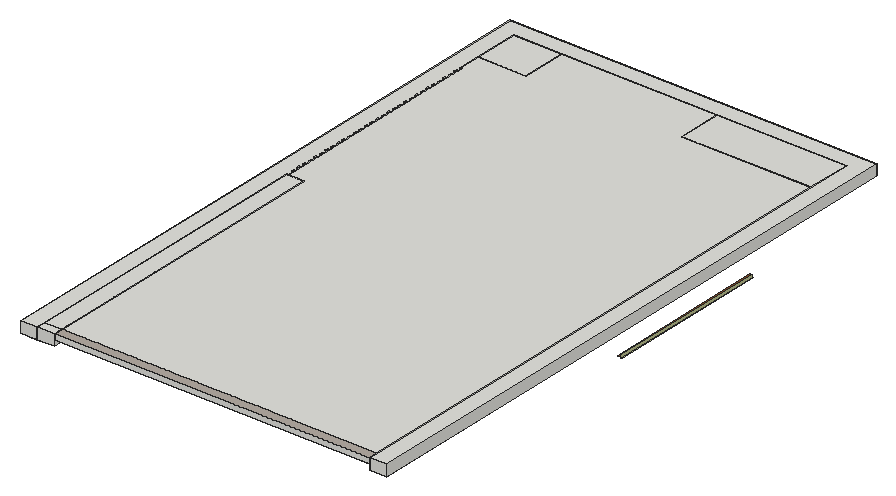
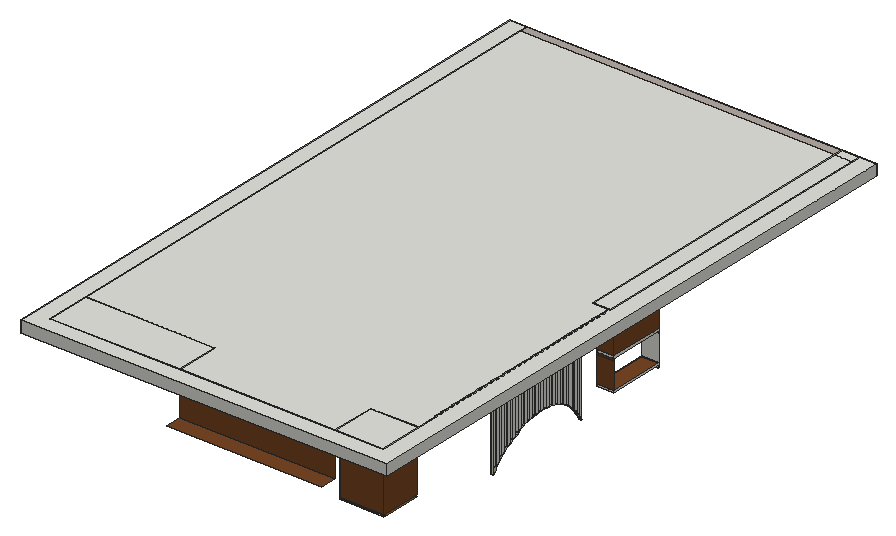
# SketchUp Ruby script. Lengths in inches.
U = 1.inch
M = Sketchup.active_model
def pt(a) = Geom::Point3d.new(a.map { |v| v * U })
def face(e, loops, mat)
  f = e.add_face(loops[0].map { |a| pt(a) })
  loops[1..].each { |l| e.add_face(l.map { |a| pt(a) }).erase! }
  f.material = f.back_material = mat if mat
  f
end
# faces: each face lists its corners as indices into pts; further lists are holes
def faces(e, pts, list, mat = nil) = list.each { |f| face(e, (f[0].is_a?(Array) ? f : [f]).map { |l| l.map { |i| pts[i] } }, mat) }
# xy, xz, yz: faces in a plane at the given z, y or x. An outline is a flat list of corners, or four numbers for a rectangle; further outlines are holes
def ring(l) = l.size == 4 ? [[l[0], l[1]], [l[2], l[1]], [l[2], l[3]], [l[0], l[3]]] : l.each_slice(2).to_a
def flat(e, list, mat, &to3) = list.each { |f| face(e, (f[0].is_a?(Array) ? f : [f]).map { |l| ring(l).map { |u, v| to3.(u, v) } }, mat) }
def xy(e, z, list, mat = nil) = flat(e, list, mat) { |x, y| [x, y, z] }
def xz(e, y, list, mat = nil) = flat(e, list, mat) { |x, z| [x, y, z] }
def yz(e, x, list, mat = nil) = flat(e, list, mat) { |y, z| [x, y, z] }
def lines(e, pts, list) = list.each { |a, b| e.add_line(pt(pts[a]), pt(pts[b])) }
# prism: a flat outline (further loops are holes) pulled along v
def prism(e, loops, v, mat = nil)
  f = face(e, loops, mat); d = Geom::Vector3d.new(v.map { |x| x * U })
  f.pushpull(f.normal.samedirection?(d) ? d.length : -d.length)
end
def box(e, o, s, mat = nil) = prism(e, [[o, [o[0] + s[0], o[1], o[2]], [o[0] + s[0], o[1] + s[1], o[2]], [o[0], o[1] + s[1], o[2]]]], [0, 0, s[2]], mat)
def at(x, y, z, deg = 0) = Geom::Transformation.translation(pt([x, y, z])) * Geom::Transformation.rotation(ORIGIN, Z_AXIS, deg.degrees)
def axes(o, x, y, z) = Geom::Transformation.new([*x, 0, *y, 0, *z, 0, *pt(o).to_a, 1])
def part(name) = M.definitions.add(name)
# library, detail: a bought-in or finely detailed component or shape, given as its bounding box
def library(name, o, s) = part(name).tap { |d| box(d.entities, o, s) }
def detail(e, o, s) = box(e.add_group.entities, o, s)
def put(e, d, t, mat = nil) = e.add_instance(d, t).tap { |i| i.material = mat if mat }
def group(e, t, mat = nil) = e.add_group.tap { |g| g.transformation = t; g.material = mat if mat }.entities
root = M.entities
M.materials.add("Emissive").color = [188, 193, 143]
M.materials.add("Generic\#1").color = [209, 204, 204]
M.materials.add("Tiles L01 200cm").color = [180, 171, 163]
M.materials.add("[Wood Veneer 01]").color = [120, 70, 37]
c1 = library("Books 297 001 004",[-3.55,-2.96,-0.03],[7.44,5.56,6.72])
c2 = library("Tlon Light 1950 Ceiling 152 010",[-38.39,-38.39,-3.78],[76.78,76.78,3.41])
xy(root,83.25,[[9,135.6,18.5,135.64]])
xy(root,84.82,[[9,135.65,10,165.95]],"Emissive")
xy(root,84.82,[[10,135.65,18.5,165.95]],"[Wood Veneer 01]")
xy(root,85.69,[[9,135.6,18.5,135.64]])
xy(root,85.69,[[9,135.64,18.5,165.95]],"[Wood Veneer 01]")
xy(root,92,[[10.03,319.1875,34,320.1875]],"Emissive")
xy(root,92,[[10.03,298.1875,34,319.1875]],"[Wood Veneer 01]")
xy(root,93,[[10,298.1875,34,320.1875]],"[Wood Veneer 01]")
xy(root,97.62,[[8.625,217.16,9.8125,217.65],[8.625,217.65,9.8125,217.68]],"Emissive")
xy(root,99.15,[[188.1875,170.86,189,259.23]],"Emissive")
xy(root,100.27,[[187.125,169.73,188.1875,259.23]],"[Wood Veneer 01]")
xy(root,101.13,[[9,135.6,10,165.91]],"Emissive")
xy(root,101.13,[[10,135.6,18.5,165.91]],"[Wood Veneer 01]")
xy(root,102.44,[[9,135.6,18.5,165.91]],"[Wood Veneer 01]")
xy(root,102.58,[[35,322.1875,119,331.1875]],"[Wood Veneer 01]")
xy(root,115,[[10,319.1875,34,320.1875]],"Emissive")
xy(root,115,[[10,298.1875,34,319.1875]],"[Wood Veneer 01]")
xy(root,116,[[9,298.1875,35,322.1875]])
xy(root,117.41,[[9,135.78,10,166.08]],"Emissive")
xy(root,117.41,[[10,135.78,18.5,166.08]],"[Wood Veneer 01]")
xy(root,120,[[0,0,0,331.1875,198,331.1875,198,0,189,0,189,322.1875,9,322.1875,9,285.93,9.8125,285.93,9.8125,283.51,9,283.51,9,282.14,9.8125,282.14,9.8125,279.71,9,279.71,9,278.35,9.8125,278.35,9.8125,275.92,9,275.92,9,274.56,9.8125,274.56,9.8125,272.13,9,272.13,9,270.77,9.8125,270.77,9.8125,268.34,9,268.34,9,266.97,9.8125,266.97,9.8125,264.55,9,264.55,9,263.18,9.8125,263.18,9.8125,260.76,9,260.76,9,259.39,9.8125,259.39,9.8125,256.96,9,256.96,9,255.6,9.8125,255.6,9.8125,253.17,9,253.17,9,251.81,9.8125,251.81,9.8125,249.38,9,249.38,9,248.02,9.8125,248.02,9.8125,245.59,9,245.59,9,244.22,9.8125,244.22,9.8125,241.8,9,241.8,9,240.43,9.8125,240.43,9.8125,238.01,9,238.01,9,236.64,9.8125,236.64,9.8125,234.21,9,234.21,9,232.85,9.8125,232.85,9.8125,230.42,9,230.42,9,229.06,9.8125,229.06,9.8125,226.63,9,226.63,9,225.27,9.8125,225.27,9.8125,222.84,9,222.84,9,221.47,9.8125,221.47,9.8125,219.05,9,219.05,9,217.68,9.8125,217.68,9.8125,215.26,9,215.26,9,213.89,9.8125,213.89,9.8125,211.46,9,211.46,9,210.1,9.8125,210.1,9.8125,207.67,9,207.67,9,206.31,9.8125,206.31,9.8125,203.88,9,203.88,9,202.52,9.9375,202.52,9.9375,200.09,9,200.09,9,198.72,9.9375,198.72,9.9375,196.3,9,196.3,9,194.93,9.9375,194.93,9.9375,192.51,9,192.51,9,191.14,9.9375,191.14,9.9375,188.71,9,188.71,9,187.35,9.9375,187.35,9.9375,184.92,9,184.92,9,183.56,9.9375,183.56,9.9375,181.13,9,181.13,9,179.77,9.9375,179.77,9.9375,177.34,9,177.34,9,175.97,9.9375,175.97,9.9375,173.55,9,173.55,9,172.18,9.9375,172.18,9.9375,168.67,9,168.67,9,0],[9,0,18.5,133.1875],[9,133.1875,18.5,168.67],[9,298.1875,35,322.1875],[119,298.1875,189,322.1875]])
xy(root,120,[[[18.5,133.1875,18.5,168.67,9.9375,168.67,9.9375,172.18,9,172.18,9,173.55,9.9375,173.55,9.9375,175.97,9,175.97,9,177.34,9.9375,177.34,9.9375,179.77,9,179.77,9,181.13,9.9375,181.13,9.9375,183.56,9,183.56,9,184.92,9.9375,184.92,9.9375,187.35,9,187.35,9,188.71,9.9375,188.71,9.9375,191.14,9,191.14,9,192.51,9.9375,192.51,9.9375,194.93,9,194.93,9,196.3,9.9375,196.3,9.9375,198.72,9,198.72,9,200.09,9.9375,200.09,9.9375,202.52,9,202.52,9,203.88,9.8125,203.88,9.8125,206.31,9,206.31,9,207.67,9.8125,207.67,9.8125,210.1,9,210.1,9,211.46,9.8125,211.46,9.8125,213.89,9,213.89,9,215.26,9.8125,215.26,9.8125,217.68,9,217.68,9,219.05,9.8125,219.05,9.8125,221.47,9,221.47,9,222.84,9.8125,222.84,9.8125,225.27,9,225.27,9,226.63,9.8125,226.63,9.8125,229.06,9,229.06,9,230.42,9.8125,230.42,9.8125,232.85,9,232.85,9,234.21,9.8125,234.21,9.8125,236.64,9,236.64,9,238.01,9.8125,238.01,9.8125,240.43,9,240.43,9,241.8,9.8125,241.8,9.8125,244.22,9,244.22,9,245.59,9.8125,245.59,9.8125,248.02,9,248.02,9,249.38,9.8125,249.38,9.8125,251.81,9,251.81,9,253.17,9.8125,253.17,9.8125,255.6,9,255.6,9,256.96,9.8125,256.96,9.8125,259.39,9,259.39,9,260.76,9.8125,260.76,9.8125,263.18,9,263.18,9,264.55,9.8125,264.55,9.8125,266.97,9,266.97,9,268.34,9.8125,268.34,9.8125,270.77,9,270.77,9,272.13,9.8125,272.13,9.8125,274.56,9,274.56,9,275.92,9.8125,275.92,9.8125,278.35,9,278.35,9,279.71,9.8125,279.71,9.8125,282.14,9,282.14,9,283.51,9.8125,283.51,9.8125,285.93,9,285.93,9,298.1875,35,298.1875,35,322.1875,119,322.1875,119,298.1875,189,298.1875,189,133.1875],[30.9375,166.1875,163.4375,277.125]]],"Generic\#1")
xy(root,123,[[18.5,0,189,133.1875],[[18.5,133.1875,189,133.1875,189,298.1875,119,298.1875,119,322.1875,35,322.1875,35,298.1875,9,298.1875,9,285.93,9.8125,285.93,9.8125,283.51,9,283.51,9,282.14,9.8125,282.14,9.8125,279.71,9,279.71,9,278.35,9.8125,278.35,9.8125,275.92,9,275.92,9,274.56,9.8125,274.56,9.8125,272.13,9,272.13,9,270.77,9.8125,270.77,9.8125,268.34,9,268.34,9,266.97,9.8125,266.97,9.8125,264.55,9,264.55,9,263.18,9.8125,263.18,9.8125,260.76,9,260.76,9,259.39,9.8125,259.39,9.8125,256.96,9,256.96,9,255.6,9.8125,255.6,9.8125,253.17,9,253.17,9,251.81,9.8125,251.81,9.8125,249.38,9,249.38,9,248.02,9.8125,248.02,9.8125,245.59,9,245.59,9,244.22,9.8125,244.22,9.8125,241.8,9,241.8,9,240.43,9.8125,240.43,9.8125,238.01,9,238.01,9,236.64,9.8125,236.64,9.8125,234.21,9,234.21,9,232.85,9.8125,232.85,9.8125,230.42,9,230.42,9,229.06,9.8125,229.06,9.8125,226.63,9,226.63,9,225.27,9.8125,225.27,9.8125,222.84,9,222.84,9,221.47,9.8125,221.47,9.8125,219.05,9,219.05,9,217.68,9.8125,217.68,9.8125,215.26,9,215.26,9,213.89,9.8125,213.89,9.8125,211.46,9,211.46,9,210.1,9.8125,210.1,9.8125,207.67,9,207.67,9,206.31,9.8125,206.31,9.8125,203.88,9,203.88,9,202.52,9.9375,202.52,9.9375,200.09,9,200.09,9,198.72,9.9375,198.72,9.9375,196.3,9,196.3,9,194.93,9.9375,194.93,9.9375,192.51,9,192.51,9,191.14,9.9375,191.14,9.9375,188.71,9,188.71,9,187.35,9.9375,187.35,9.9375,184.92,9,184.92,9,183.56,9.9375,183.56,9.9375,181.13,9,181.13,9,179.77,9.9375,179.77,9.9375,177.34,9,177.34,9,175.97,9.9375,175.97,9.9375,173.55,9,173.55,9,172.18,9.9375,172.18,9.9375,168.67,18.5,168.67],[28.1875,164.375,165.25,279.875]]])
xy(root,123,[[28.1875,164.375,163.4375,166.1875],[163.4375,164.375,165.25,279.875],[28.1875,166.1875,30.9375,277.125],[28.1875,277.125,163.4375,279.875]],"Emissive")
xy(root,124,[[28.1875,164.375,165.25,279.875]],"Generic\#1")
xy(root,126,[[0,0,9,0,9,168.67,9.9375,168.67,9.9375,172.18,9,172.18,9,173.55,9.9375,173.55,9.9375,175.97,9,175.97,9,177.34,9.9375,177.34,9.9375,179.77,9,179.77,9,181.13,9.9375,181.13,9.9375,183.56,9,183.56,9,184.92,9.9375,184.92,9.9375,187.35,9,187.35,9,188.71,9.9375,188.71,9.9375,191.14,9,191.14,9,192.51,9.9375,192.51,9.9375,194.93,9,194.93,9,196.3,9.9375,196.3,9.9375,198.72,9,198.72,9,200.09,9.9375,200.09,9.9375,202.52,9,202.52,9,203.88,9.8125,203.88,9.8125,206.31,9,206.31,9,207.67,9.8125,207.67,9.8125,210.1,9,210.1,9,211.46,9.8125,211.46,9.8125,213.89,9,213.89,9,215.26,9.8125,215.26,9.8125,217.68,9,217.68,9,219.05,9.8125,219.05,9.8125,221.47,9,221.47,9,222.84,9.8125,222.84,9.8125,225.27,9,225.27,9,226.63,9.8125,226.63,9.8125,229.06,9,229.06,9,230.42,9.8125,230.42,9.8125,232.85,9,232.85,9,234.21,9.8125,234.21,9.8125,236.64,9,236.64,9,238.01,9.8125,238.01,9.8125,240.43,9,240.43,9,241.8,9.8125,241.8,9.8125,244.22,9,244.22,9,245.59,9.8125,245.59,9.8125,248.02,9,248.02,9,249.38,9.8125,249.38,9.8125,251.81,9,251.81,9,253.17,9.8125,253.17,9.8125,255.6,9,255.6,9,256.96,9.8125,256.96,9.8125,259.39,9,259.39,9,260.76,9.8125,260.76,9.8125,263.18,9,263.18,9,264.55,9.8125,264.55,9.8125,266.97,9,266.97,9,268.34,9.8125,268.34,9.8125,270.77,9,270.77,9,272.13,9.8125,272.13,9.8125,274.56,9,274.56,9,275.92,9.8125,275.92,9.8125,278.35,9,278.35,9,279.71,9.8125,279.71,9.8125,282.14,9,282.14,9,283.51,9.8125,283.51,9.8125,285.93,9,285.93,9,322.1875,189,322.1875,189,0,198,0,198,331.1875,0,331.1875],[9,0,18.5,5.08],[18.5,5.08,189,5.08,189,298.1875,119,298.1875,119,322.1875,35,322.1875,35,298.1875,9,298.1875,9,285.93,9.8125,285.93,9.8125,283.51,9,283.51,9,282.14,9.8125,282.14,9.8125,279.71,9,279.71,9,278.35,9.8125,278.35,9.8125,275.92,9,275.92,9,274.56,9.8125,274.56,9.8125,272.13,9,272.13,9,270.77,9.8125,270.77,9.8125,268.34,9,268.34,9,266.97,9.8125,266.97,9.8125,264.55,9,264.55,9,263.18,9.8125,263.18,9.8125,260.76,9,260.76,9,259.39,9.8125,259.39,9.8125,256.96,9,256.96,9,255.6,9.8125,255.6,9.8125,253.17,9,253.17,9,251.81,9.8125,251.81,9.8125,249.38,9,249.38,9,248.02,9.8125,248.02,9.8125,245.59,9,245.59,9,244.22,9.8125,244.22,9.8125,241.8,9,241.8,9,240.43,9.8125,240.43,9.8125,238.01,9,238.01,9,236.64,9.8125,236.64,9.8125,234.21,9,234.21,9,232.85,9.8125,232.85,9.8125,230.42,9,230.42,9,229.06,9.8125,229.06,9.8125,226.63,9,226.63,9,225.27,9.8125,225.27,9.8125,222.84,9,222.84,9,221.47,9.8125,221.47,9.8125,219.05,9,219.05,9,217.68,9.8125,217.68,9.8125,215.26,9,215.26,9,213.89,9.8125,213.89,9.8125,211.46,9,211.46,9,210.1,9.8125,210.1,9.8125,207.67,9,207.67,9,206.31,9.8125,206.31,9.8125,203.88,9,203.88,9,202.52,9.9375,202.52,9.9375,200.09,9,200.09,9,198.72,9.9375,198.72,9.9375,196.3,9,196.3,9,194.93,9.9375,194.93,9.9375,192.51,9,192.51,9,191.14,9.9375,191.14,9.9375,188.71,9,188.71,9,187.35,9.9375,187.35,9.9375,184.92,9,184.92,9,183.56,9.9375,183.56,9.9375,181.13,9,181.13,9,179.77,9.9375,179.77,9.9375,177.34,9,177.34,9,175.97,9.9375,175.97,9.9375,173.55,9,173.55,9,172.18,9.9375,172.18,9.9375,168.67,18.5,168.67],[9,5.08,18.5,168.67],[9,298.1875,35,322.1875],
  [119,298.1875,189,322.1875]])
xy(root,126,[[18.5,0,189,5.08]],"Tiles L01 200cm")
xz(root,0,[[0,120,9,126],[9,120,18.5,126],[189,120,198,126],[18.5,123,189,126]])
xz(root,133.1875,[[18.5,120,189,123]])
xz(root,135.6,[[9,83.25,18.5,85.69],[9,100.13,18.5,101.13],[9,101.13,18.5,102.44],[9,102.44,18.5,102.57]])
xz(root,135.64,[[9,83.25,18.5,85.69]])
xz(root,135.65,[[9,83.25,18.5,84.82]])
xz(root,164.375,[[28.1875,123,165.25,124]],"Emissive")
xz(root,165.91,[[9,101.13,18.5,102.44],[9,102.44,18.5,102.57]])
xz(root,165.91,[[9,100.13,18.5,101.13]],"[Wood Veneer 01]")
xz(root,165.95,[[9,84.82,18.5,85.69]])
xz(root,166.1875,[[30.9375,120,163.4375,123]])
xz(root,168.67,[[9,120,9.9375,126],[9.9375,120,18.5,123],[9.9375,123,18.5,126]])
xz(root,172.18,[[9,120,9.9375,123],[9,123,9.9375,126]])
xz(root,173.55,[[9,120,9.9375,123],[9,123,9.9375,126]])
xz(root,175.97,[[9,120,9.9375,123],[9,123,9.9375,126]])
xz(root,177.34,[[9,120,9.9375,123],[9,123,9.9375,126]])
xz(root,179.77,[[9,120,9.9375,123],[9,123,9.9375,126]])
xz(root,181.13,[[9,120,9.9375,123],[9,123,9.9375,126]])
xz(root,183.56,[[9,120,9.9375,123],[9,123,9.9375,126]])
xz(root,184.92,[[9,120,9.9375,123],[9,123,9.9375,126]])
xz(root,187.35,[[9,120,9.9375,123],[9,123,9.9375,126]])
xz(root,188.71,[[9,81.82,9.9375,120],[9,120,9.9375,123],[9,123,9.9375,126]])
xz(root,191.14,[[9,85.88,9.9375,120],[9,120,9.9375,123],[9,123,9.9375,126]])
xz(root,191.14,[[8.625,85.875,9.9375,85.88]],"Emissive")
xz(root,192.51,[[9,87.65,9.9375,120],[9,120,9.9375,123],[9,123,9.9375,126]])
xz(root,194.93,[[9,90.26,9.9375,120],[9,120,9.9375,123],[9,123,9.9375,126]])
xz(root,196.3,[[9,91.4375,9.9375,120],[9,120,9.9375,123],[9,123,9.9375,126]])
xz(root,198.72,[[9,93.24,9.9375,120],[9,120,9.9375,123],[9,123,9.9375,126]])
xz(root,200.09,[[9,94.09,9.9375,120],[9,120,9.9375,123],[9,123,9.9375,126]])
xz(root,202.52,[[9,95.34,9.9375,120],[9,120,9.9375,123],[9,123,9.9375,126]])
xz(root,203.88,[[9,95.9,9.8125,120],[9,120,9.8125,123],[9,123,9.8125,126]])
xz(root,206.31,[[9,96.72,9.8125,120],[9,120,9.8125,123],[9,123,9.8125,126]])
xz(root,207.67,[[9,97.11,9.8125,120],[9,120,9.8125,123],[9,123,9.8125,126]])
xz(root,210.1,[[9,97.54,9.8125,120],[9,120,9.8125,123],[9,123,9.8125,126]])
xz(root,211.46,[[9,97.69,9.8125,120],[9,120,9.8125,123],[9,123,9.8125,126]])
xz(root,213.89,[[9,97.82,9.8125,120],[9,120,9.8125,123],[9,123,9.8125,126]])
xz(root,215.26,[[9,97.76,9.8125,120],[9,120,9.8125,123],[9,123,9.8125,126]])
xz(root,217.68,[[9,97.62,9.8125,120],[9,120,9.8125,123],[9,123,9.8125,126]])
xz(root,219.05,[[9,97.57,9.8125,120],[9,120,9.8125,123],[9,123,9.8125,126]])
xz(root,221.47,[[9,97.27,9.8125,120],[9,120,9.8125,123],[9,123,9.8125,126]])
xz(root,222.84,[[9,96.98,9.8125,120],[9,120,9.8125,123],[9,123,9.8125,126]])
xz(root,225.27,[[9,96.66,9.8125,120],[9,120,9.8125,123],[9,123,9.8125,126]])
xz(root,226.63,[[9,96.31,9.8125,120],[9,120,9.8125,123],[9,123,9.8125,126]])
xz(root,229.06,[[9,95.27,9.8125,120],[9,120,9.8125,123],[9,123,9.8125,126]])
xz(root,230.42,[[9,94.42,9.8125,120],[9,120,9.8125,123],[9,123,9.8125,126]])
xz(root,232.85,[[9,92.875,9.8125,120],[9,120,9.8125,123],[9,123,9.8125,126]])
xz(root,234.21,[[9,92.35,9.8125,120],[9,120,9.8125,123],[9,123,9.8125,126]])
xz(root,236.64,[[9,91.21,9.8125,120],[9,120,9.8125,123],[9,123,9.8125,126]])
xz(root,238.01,[[9,90.48,9.8125,120],[9,120,9.8125,123],[9,123,9.8125,126]])
xz(root,240.43,[[9,88.9,9.8125,120],[9,120,9.8125,123],[9,123,9.8125,126]])
xz(root,241.8,[[9,87.8,9.8125,120],[9,120,9.8125,123],[9,123,9.8125,126]])
xz(root,244.22,[[9,85.6,9.8125,120],[9,120,9.8125,123],[9,123,9.8125,126]])
xz(root,245.59,[[9,84.16,9.8125,120],[9,120,9.8125,123],[9,123,9.8125,126]])
xz(root,248.02,[[9,80.92,9.8125,120],[9,120,9.8125,123],[9,123,9.8125,126]])
xz(root,249.38,[[9,120,9.8125,123],[9,123,9.8125,126]])
xz(root,251.81,[[9,120,9.8125,123],[9,123,9.8125,126]])
xz(root,253.17,[[9,120,9.8125,123],[9,123,9.8125,126]])
xz(root,255.6,[[9,120,9.8125,123],[9,123,9.8125,126]])
xz(root,256.96,[[9,120,9.8125,123],[9,123,9.8125,126]])
xz(root,259.39,[[9,120,9.8125,123],[9,123,9.8125,126]])
xz(root,260.76,[[9,120,9.8125,123],[9,123,9.8125,126]])
xz(root,263.18,[[9,120,9.8125,123],[9,123,9.8125,126]])
xz(root,264.55,[[9,120,9.8125,123],[9,123,9.8125,126]])
xz(root,266.97,[[9,120,9.8125,123],[9,123,9.8125,126]])
xz(root,268.34,[[9,120,9.8125,123],[9,123,9.8125,126]])
xz(root,270.77,[[9,120,9.8125,123],[9,123,9.8125,126]])
xz(root,272.13,[[9,120,9.8125,123],[9,123,9.8125,126]])
xz(root,274.56,[[9,120,9.8125,123],[9,123,9.8125,126]])
xz(root,275.92,[[9,120,9.8125,123],[9,123,9.8125,126]])
xz(root,277.125,[[30.9375,120,163.4375,123]],"Generic\#1")
xz(root,278.35,[[9,120,9.8125,123],[9,123,9.8125,126]])
xz(root,279.71,[[9,120,9.8125,123],[9,123,9.8125,126]])
xz(root,279.875,[[28.1875,123,165.25,124]],"Emissive")
xz(root,282.14,[[9,120,9.8125,123],[9,123,9.8125,126]])
xz(root,283.51,[[9,120,9.8125,123],[9,123,9.8125,126]])
xz(root,285.93,[[9,120,9.8125,123],[9,123,9.8125,126]])
xz(root,298.1875,[[9,120,35,123],[119,120,189,123],[9,123,35,126],[119,123,189,126]])
xz(root,298.1875,[[9,116,35,120]],"[Wood Veneer 01]")
xz(root,320.1875,[[10,93,34,115]],"[Wood Veneer 01]")
xz(root,322.1875,[[9,116,35,120],[9,120,35,126],[35,120,119,123],[119,120,189,126],[35,123,119,126]])
xz(root,322.1875,[[35,102.58,119,120]],"[Wood Veneer 01]")
xz(root,331.1875,[[0,120,198,126]])
yz(root,0,[[0,120,331.1875,126]])
yz(root,9,[[135.6,83.25,135.64,85.69],[135.64,83.25,135.65,83.25,135.64,85.69],[135.65,83.25,135.64,85.69,165.95,85.69,165.95,84.82,135.65,84.82],[245.59,84.16,245.59,120,244.22,120,244.22,85.6,245.31,84.5],[191.14,85.88,192.51,87.65,192.51,120,191.14,120],
  [241.8,87.8,241.8,120,240.43,120,240.43,88.9,240.51,88.85],[194.93,90.26,196.3,91.4375,196.3,120,194.93,120],[238.01,90.48,238.01,120,236.64,120,236.64,91.21,237.78,90.625],[234.21,92.35,234.21,120,232.85,120,232.85,92.875],[198.72,93.24,199.49,93.76,200.09,94.09,200.09,120,198.72,120],
  [230.42,94.42,230.42,120,229.06,120,229.06,95.27,229.5,95.03,230.32,94.49],[202.52,95.34,203.88,95.9,203.88,120,202.52,120],[226.63,96.31,226.63,120,225.27,120,225.27,96.66,225.87,96.53],[206.31,96.72,207.67,97.11,207.67,120,206.31,120],[222.84,96.98,222.84,120,221.47,120,221.47,97.27,221.53,97.26,222,97.16,222.48,97.0625],
  [210.1,97.54,210.66,97.64,211.46,97.69,211.46,120,210.1,120],[219.05,97.57,219.05,120,217.68,120,217.68,97.62,218.14,97.61,218.625,97.59],[215.26,97.76,215.26,120,213.89,120,213.89,97.82],[135.6,101.13,165.91,102.44],[298.1875,116,322.1875,120],
  [0,120,5.08,126],[5.08,120,168.67,126],[172.18,120,173.55,123],[175.97,120,177.34,123],[179.77,120,181.13,123],
  [183.56,120,184.92,123],[187.35,120,188.71,123],[191.14,120,192.51,123],[194.93,120,196.3,123],[198.72,120,200.09,123],
  [202.52,120,203.88,123],[206.31,120,207.67,123],[210.1,120,211.46,123],[213.89,120,215.26,123],[217.68,120,219.05,123],
  [221.47,120,222.84,123],[225.27,120,226.63,123],[229.06,120,230.42,123],[232.85,120,234.21,123],[236.64,120,238.01,123],
  [240.43,120,241.8,123],[244.22,120,245.59,123],[248.02,120,249.38,123],[251.81,120,253.17,123],[255.6,120,256.96,123],
  [259.39,120,260.76,123],[263.18,120,264.55,123],[266.97,120,268.34,123],[270.77,120,272.13,123],[274.56,120,275.92,123],
  [278.35,120,279.71,123],[282.14,120,283.51,123],[285.93,120,287.3,123],[287.3,120,298.1875,123],[298.1875,120,322.1875,126],
  [172.18,123,173.55,126],[175.97,123,177.34,126],[179.77,123,181.13,126],[183.56,123,184.92,126],[187.35,123,188.71,126],
  [191.14,123,192.51,126],[194.93,123,196.3,126],[198.72,123,200.09,126],[202.52,123,203.88,126],[206.31,123,207.67,126],
  [210.1,123,211.46,126],[213.89,123,215.26,126],[217.68,123,219.05,126],[221.47,123,222.84,126],[225.27,123,226.63,126],
  [229.06,123,230.42,126],[232.85,123,234.21,126],[236.64,123,238.01,126],[240.43,123,241.8,126],[244.22,123,245.59,126],
  [248.02,123,249.38,126],[251.81,123,253.17,126],[255.6,123,256.96,126],[259.39,123,260.76,126],[263.18,123,264.55,126],
  [266.97,123,268.34,126],[270.77,123,272.13,126],[274.56,123,275.92,126],[278.35,123,279.71,126],[282.14,123,283.51,126],
  [285.93,123,287.3,126],[287.3,123,298.1875,126]])
yz(root,9,[[135.6,102.44,165.91,102.44,165.91,102.57,166.08,117.41,135.78,117.41,135.6,102.57]],"[Wood Veneer 01]")
yz(root,9.8125,[[248.02,80.92,248.02,120,245.59,120,245.59,84.16,247.35,81.97],[244.22,85.6,244.22,120,241.8,120,241.8,87.8,243.03,86.81],[240.43,88.9,240.43,120,238.01,120,238.01,90.48],[236.64,91.21,236.64,120,234.21,120,234.21,92.35,234.89,92.1],[232.85,92.875,232.85,120,230.42,120,230.42,94.42,231.11,93.9,231.85,93.26],
  [229.06,95.27,229.06,120,226.63,120,226.63,96.31,226.82,96.25,227.74,95.91,228.63,95.5],[203.88,95.9,204.87,96.3,206.31,96.72,206.31,120,203.88,120],[225.27,96.66,225.27,120,222.84,120,222.84,96.98,222.96,96.95,223.9375,96.88,224.91,96.74],[207.67,97.11,207.73,97.125,210.1,97.54,210.1,120,207.67,120],[221.47,97.27,221.47,120,219.05,120,219.05,97.57,219.11,97.5625,219.6,97.52,220.08,97.47,220.5625,97.41,221.05,97.34],
  [217.16,97.62,217.68,97.62,217.68,120,215.26,120,215.26,97.76,216.61,97.7],[211.46,97.69,213.63,97.83,213.89,97.82,213.89,120,211.46,120],[203.88,120,206.31,123],[207.67,120,210.1,123],[211.46,120,213.89,123],
  [215.26,120,217.68,123],[219.05,120,221.47,123],[222.84,120,225.27,123],[226.63,120,229.06,123],[230.42,120,232.85,123],
  [234.21,120,236.64,123],[238.01,120,240.43,123],[241.8,120,244.22,123],[245.59,120,248.02,123],[249.38,120,251.81,123],
  [253.17,120,255.6,123],[256.96,120,259.39,123],[260.76,120,263.18,123],[264.55,120,266.97,123],[268.34,120,270.77,123],
  [272.13,120,274.56,123],[275.92,120,278.35,123],[279.71,120,282.14,123],[283.51,120,285.93,123],[203.88,123,206.31,126],
  [207.67,123,210.1,126],[211.46,123,213.89,126],[215.26,123,217.68,126],[219.05,123,221.47,126],[222.84,123,225.27,126],
  [226.63,123,229.06,126],[230.42,123,232.85,126],[234.21,123,236.64,126],[238.01,123,240.43,126],[241.8,123,244.22,126],
  [245.59,123,248.02,126],[249.38,123,251.81,126],[253.17,123,255.6,126],[256.96,123,259.39,126],[260.76,123,263.18,126],
  [264.55,123,266.97,126],[268.34,123,270.77,126],[272.13,123,274.56,126],[275.92,123,278.35,126],[279.71,123,282.14,126],
  [283.51,123,285.93,126]])
yz(root,9.9375,[[188.71,81.82,189.71,83.67,191.14,85.875,191.14,120,188.71,120],[192.51,87.65,192.75,87.96,194.78,90.13,194.93,90.26,194.93,120,192.51,120],[196.3,91.4375,197.04,92.07,198.72,93.24,198.72,120,196.3,120],[200.09,94.09,202.11,95.18,202.52,95.34,202.52,120,200.09,120],[168.67,120,172.18,123],
  [173.55,120,175.97,123],[177.34,120,179.77,123],[181.13,120,183.56,123],[184.92,120,187.35,123],[188.71,120,191.14,123],
  [192.51,120,194.93,123],[196.3,120,198.72,123],[200.09,120,202.52,123],[168.67,123,172.18,126],[173.55,123,175.97,126],
  [177.34,123,179.77,126],[181.13,123,183.56,126],[184.92,123,187.35,126],[188.71,123,191.14,126],[192.51,123,194.93,126],
  [196.3,123,198.72,126],[200.09,123,202.52,126]])
yz(root,10,[[298.1875,93,320.1875,115]],"[Wood Veneer 01]")
yz(root,18.5,[[135.64,83.25,135.65,83.25,135.64,85.69],[0,120,133.1875,123],[133.1875,120,168.67,123],[0,123,168.67,126]])
yz(root,18.5,[[135.65,83.25,135.65,84.82,165.95,84.82,165.95,85.69,135.64,85.69],[135.6,101.13,165.91,102.44]],"[Wood Veneer 01]")
yz(root,28.1875,[[164.375,123,279.875,124]],"Emissive")
yz(root,30.9375,[[166.1875,120,277.125,123]],"Generic\#1")
yz(root,34,[[298.1875,93,320.1875,115]],"[Wood Veneer 01]")
yz(root,35,[[298.1875,120,322.1875,123],[298.1875,123,322.1875,126]])
yz(root,35,[[298.1875,116,322.1875,120]],"[Wood Veneer 01]")
yz(root,119,[[298.1875,120,322.1875,123],[298.1875,123,322.1875,126]])
yz(root,163.4375,[[166.1875,120,277.125,123]],"Generic\#1")
yz(root,165.25,[[164.375,123,279.875,124]],"Emissive")
yz(root,188.1875,[[170.86,99.15,259.23,100.27]],"Emissive")
yz(root,189,[[0,120,5.08,123],[5.08,120,133.1875,123],[133.1875,120,298.1875,123],[298.1875,120,322.1875,126],[0,123,5.08,126],
  [5.08,123,298.1875,126]])
yz(root,198,[[0,120,331.1875,126]])
p = [[8.625,248.02,80.92],[9,248.02,80.92],[9.8125,248.02,80.92],[9.8125,247.35,81.97],[8.625,247.35,81.97],[9,188.71,81.82],
  [9,188.46,81.35],[8.625,188.46,81.35],[8.625,188.71,81.82],[8.625,189.71,83.67],[9.9375,189.71,83.67],[9.9375,188.71,81.82],
  [9.8125,245.59,84.16],[9,245.59,84.16],[8.625,245.59,84.16],[9,135.65,83.25],[9,135.64,85.69],[18.5,135.64,85.69],
  [18.5,135.65,83.25],[8.625,191.14,85.875],[9.9375,191.14,85.875],[9,245.31,84.5],[8.625,245.31,84.5],[9,244.22,85.6],
  [8.625,244.22,85.6],[9.8125,244.22,85.6],[9.8125,243.03,86.81],[8.625,243.03,86.81],[9,135.6,100.13],[18.5,135.6,100.13],
  [9,165.91,100.13],[9,165.95,85.69],[18.5,165.95,85.69],[18.5,165.91,100.13],[9,192.51,87.65],[9,191.14,85.88],
  [8.625,191.14,85.88],[8.625,192.51,87.65],[9.8125,241.8,87.8],[9,241.8,87.8],[8.625,241.8,87.8],[8.625,192.75,87.96],
  [9.9375,192.75,87.96],[9.9375,192.51,87.65],[9,240.51,88.85],[8.625,240.51,88.85],[8.625,194.78,90.13],[9.9375,194.78,90.13],
  [8.625,240.43,88.9],[9,240.43,88.9],[9.8125,240.43,88.9],[9.8125,238.01,90.48],[9,238.01,90.48],[8.625,238.01,90.48],
  [8.625,194.93,90.26],[9,194.93,90.26],[9.9375,194.93,90.26],[9,196.3,91.4375],[8.625,196.3,91.4375],[9,237.78,90.625],
  [8.625,237.78,90.625],[9,236.64,91.21],[8.625,236.64,91.21],[9.8125,236.64,91.21],[9.8125,234.89,92.1],[8.625,234.89,92.1],
  [8.625,197.04,92.07],[9.9375,197.04,92.07],[9.9375,196.3,91.4375],[8.625,198.72,93.24],[9,198.72,93.24],[9.9375,198.72,93.24],
  [9.8125,234.21,92.35],[9,234.21,92.35],[8.625,234.21,92.35],[9,232.85,92.875],[8.625,232.85,92.875],[9.8125,232.85,92.875],
  [9.8125,231.85,93.26],[8.625,231.85,93.26],[9,199.49,93.76],[8.625,199.49,93.76],[9.8125,231.11,93.9],[8.625,231.11,93.9],
  [9,200.09,94.09],[8.625,200.09,94.09],[9.8125,230.42,94.42],[9,230.42,94.42],[8.625,230.42,94.42],[8.625,202.11,95.18],
  [9.9375,202.11,95.18],[9.9375,200.09,94.09],[9,230.32,94.49],[8.625,230.32,94.49],[9,229.5,95.03],[8.625,229.5,95.03],
  [9,229.06,95.27],[8.625,229.06,95.27],[8.625,202.52,95.34],[9,202.52,95.34],[9.9375,202.52,95.34],[9,203.88,95.9],
  [8.625,203.88,95.9],[9.8125,229.06,95.27],[9.8125,228.63,95.5],[8.625,228.63,95.5],[9.8125,227.74,95.91],[8.625,227.74,95.91],
  [8.625,204.87,96.3],[9.8125,204.87,96.3],[9.8125,203.88,95.9],[9.8125,226.82,96.25],[8.625,226.82,96.25],[8.625,206.31,96.72],
  [9,206.31,96.72],[9.8125,206.31,96.72],[9,226.63,96.31],[9,225.87,96.53],[8.625,225.87,96.53],[8.625,226.63,96.31],
  [9.8125,226.63,96.31],[9,225.27,96.66],[8.625,225.27,96.66],[9,207.67,97.11],[8.625,207.67,97.11],[8.625,224.91,96.74],
  [9.8125,224.91,96.74],[9.8125,223.9375,96.88],[8.625,223.9375,96.88],[9.8125,225.27,96.66],[9.8125,222.96,96.95],[8.625,222.96,96.95],
  [9,222.84,96.98],[9,222.48,97.0625],[8.625,222.48,97.0625],[8.625,222.84,96.98],[9.8125,222.84,96.98],[8.625,207.73,97.125],
  [9.8125,207.73,97.125],[9.8125,207.67,97.11],[8.625,210.1,97.54],[9,210.1,97.54],[9.8125,210.1,97.54],[9,222,97.16],
  [8.625,222,97.16],[9,221.53,97.26],[8.625,221.53,97.26],[8.625,221.05,97.34],[9.8125,221.05,97.34],[9.8125,220.5625,97.41],
  [8.625,220.5625,97.41],[8.625,221.47,97.27],[9,221.47,97.27],[9.8125,221.47,97.27],[9.8125,220.08,97.47],[8.625,220.08,97.47],
  [9,210.66,97.64],[8.625,210.66,97.64],[8.625,219.6,97.52],[9.8125,219.6,97.52],[9.8125,219.11,97.5625],[8.625,219.11,97.5625],
  [9,211.46,97.69],[8.625,211.46,97.69],[8.625,217.16,97.62],[9.8125,217.16,97.62],[9.8125,216.61,97.7],[8.625,216.61,97.7],
  [9,218.14,97.61],[9,217.68,97.62],[8.625,217.68,97.62],[8.625,218.14,97.61],[9,218.625,97.59],[8.625,218.625,97.59],
  [9,219.05,97.57],[8.625,219.05,97.57],[9.8125,219.05,97.57],[8.625,213.63,97.83],[9.8125,213.63,97.83],[9.8125,211.46,97.69],
  [9.8125,215.26,97.76],[9,215.26,97.76],[8.625,215.26,97.76],[8.625,213.89,97.82],[9,213.89,97.82],[9.8125,213.89,97.82],
  [9,135.6,102.57],[9,135.78,117.41],[10,135.78,117.41],[18.5,135.78,117.41],[18.5,135.6,102.57],[9,166.08,117.41],
  [9,165.91,102.57],[18.5,165.91,102.57],[18.5,166.08,117.41],[10,166.08,117.41]]
faces(root,p,[[0,1,2,3,4],[5,6,7,8],[9,10,11,5,8],[4,3,12,13,14],[19,20,10,9],[13,21,22,14],[21,23,24,22],[24,23,25,26,27],
  [34,35,36,37],[27,26,38,39,40],[41,42,43,34,37],[39,44,45,40],[46,47,42,41],[48,49,50,51,52,53],[44,49,48,45],[54,55,56,47,46],
  [57,55,54,58],[52,59,60,53],[59,61,62,60],[62,61,63,64,65],[66,67,68,57,58],[69,70,71,67,66],[65,64,72,73,74],[73,75,76,74],
  [76,75,77,78,79],[80,70,69,81],[79,78,82,83],[84,80,81,85],[83,82,86,87,88],[89,90,91,84,85],[87,92,93,88],[92,94,95,93],
  [94,96,97,95],[98,99,100,90,89],[101,99,98,102],[97,96,103,104,105],[105,104,106,107],[108,109,110,101,102],[107,106,111,112],[113,114,115,109,108],
  [116,117,118,119],[112,111,120,116,119],[117,121,122,118],[123,114,113,124],[125,126,127,128],[122,121,129,126,125],[128,127,130,131],[132,133,134,135],
  [131,130,136,132,135],[137,138,139,123,124],[140,141,142,138,137],[133,143,144,134],[143,145,146,144],[147,148,149,150],[151,152,153,148,147],[145,152,151,146],
  [150,149,154,155],[158,159,160,161],[155,154,159,158],[164,165,166,167],[168,169,170,171],[172,168,171,173],[174,172,173,175],[161,160,176,174,175],
  [177,178,179,162,163],[167,166,180,181,182],[183,184,185,178,177],[181,184,183,182]],"Emissive")
faces(root,p,[[15,16,17,18],[16,28,29,17],[156,141,140,157],[162,156,157,163],[186,187,188,189,190]])
faces(root,p,[[30,31,32,33],[191,192,193,194,195]],"[Wood Veneer 01]")
put(root,c1,axes([16.31,306.875,93.02],[1.66,0,0],[0,1.66,0],[0,0,1.66]))
put(root,c2,axes([61.52,153.27,120.23],[0.11,0,0],[0,0.11,0],[0,0,0.11]))
put(root,c2,axes([108.64,153.27,120.23],[0.11,0,0],[0,0.11,0],[0,0,0.11]))
put(root,c2,axes([169.27,153.27,120.23],[0.11,0,0],[0,0.11,0],[0,0,0.11]))
put(root,c2,axes([169.27,208.39,120.23],[0.11,0,0],[0,0.11,0],[0,0,0.11]))
put(root,c2,axes([169.27,272.52,120.23],[0.11,0,0],[0,0.11,0],[0,0,0.11]))
put(root,c2,axes([88.76,288.73,120.23],[0.11,0,0],[0,0.11,0],[0,0,0.11]))
put(root,c2,axes([52.94,288.73,120.23],[0.11,0,0],[0,0.11,0],[0,0,0.11]))
put(root,c2,axes([19.625,243.18,120.23],[0.11,0,0],[0,0.11,0],[0,0,0.11]))
put(root,c2,axes([19.625,199.43,120.23],[0.11,0,0],[0,0.11,0],[0,0,0.11]))
